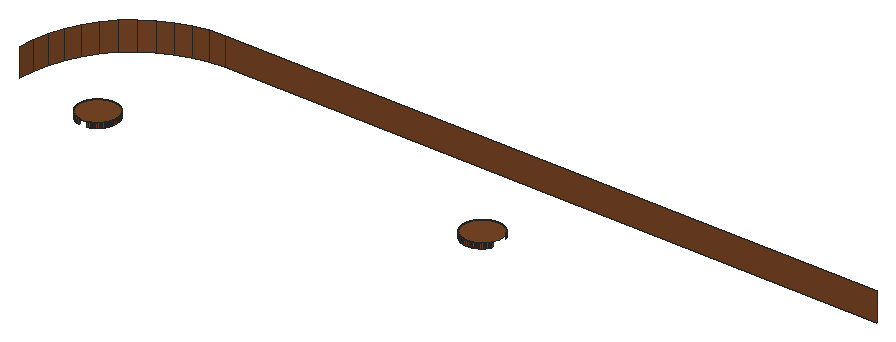
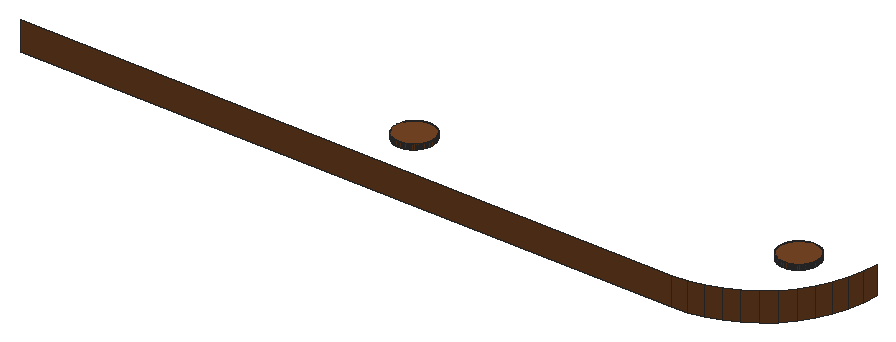
# SketchUp Ruby script. Lengths in inches.
U = 1.inch
M = Sketchup.active_model
def pt(a) = Geom::Point3d.new(a.map { |v| v * U })
def face(e, loops, mat)
  f = e.add_face(loops[0].map { |a| pt(a) })
  loops[1..].each { |l| e.add_face(l.map { |a| pt(a) }).erase! }
  f.material = f.back_material = mat if mat
  f
end
# faces: each face lists its corners as indices into pts; further lists are holes
def faces(e, pts, list, mat = nil) = list.each { |f| face(e, (f[0].is_a?(Array) ? f : [f]).map { |l| l.map { |i| pts[i] } }, mat) }
# xy, xz, yz: faces in a plane at the given z, y or x. An outline is a flat list of corners, or four numbers for a rectangle; further outlines are holes
def ring(l) = l.size == 4 ? [[l[0], l[1]], [l[2], l[1]], [l[2], l[3]], [l[0], l[3]]] : l.each_slice(2).to_a
def flat(e, list, mat, &to3) = list.each { |f| face(e, (f[0].is_a?(Array) ? f : [f]).map { |l| ring(l).map { |u, v| to3.(u, v) } }, mat) }
def xy(e, z, list, mat = nil) = flat(e, list, mat) { |x, y| [x, y, z] }
def xz(e, y, list, mat = nil) = flat(e, list, mat) { |x, z| [x, y, z] }
def yz(e, x, list, mat = nil) = flat(e, list, mat) { |y, z| [x, y, z] }
def lines(e, pts, list) = list.each { |a, b| e.add_line(pt(pts[a]), pt(pts[b])) }
# prism: a flat outline (further loops are holes) pulled along v
def prism(e, loops, v, mat = nil)
  f = face(e, loops, mat); d = Geom::Vector3d.new(v.map { |x| x * U })
  f.pushpull(f.normal.samedirection?(d) ? d.length : -d.length)
end
def box(e, o, s, mat = nil) = prism(e, [[o, [o[0] + s[0], o[1], o[2]], [o[0] + s[0], o[1] + s[1], o[2]], [o[0], o[1] + s[1], o[2]]]], [0, 0, s[2]], mat)
def at(x, y, z, deg = 0) = Geom::Transformation.translation(pt([x, y, z])) * Geom::Transformation.rotation(ORIGIN, Z_AXIS, deg.degrees)
def axes(o, x, y, z) = Geom::Transformation.new([*x, 0, *y, 0, *z, 0, *pt(o).to_a, 1])
def part(name) = M.definitions.add(name)
# library, detail: a bought-in or finely detailed component or shape, given as its bounding box
def library(name, o, s) = part(name).tap { |d| box(d.entities, o, s) }
def detail(e, o, s) = box(e.add_group.entities, o, s)
def put(e, d, t, mat = nil) = e.add_instance(d, t).tap { |i| i.material = mat if mat }
def group(e, t, mat = nil) = e.add_group.tap { |g| g.transformation = t; g.material = mat if mat }.entities
root = M.entities
M.materials.add("[Wood Veneer 01]3").color = [120, 70, 37]
xy(root,118.5,[[71.9,168,71.74,168.02,71.65,168.03,71.41,168.09,71.17,168.18,71.1,168.21,71.02,168.25,70.95,168.3,70.88,168.34,70.8125,168.39,70.75,168.44,70.68,168.5,70.62,168.55,70.5625,168.61,70.5,168.67,70.45,168.74,70.4,168.8,70.3,168.94,70.26,169.01,70.22,169.09,70.18,169.16,70.09,169.4,70.03,169.64,70.01,169.8,70,169.89,70,170.14,70.01,170.22,70.02,170.31,70.1,170.63,70.16,170.79,70.2,170.86,70.23,170.9375,70.27,171.01,70.47,171.29,70.52,171.35,70.64,171.47,70.7,171.52,70.77,171.58,70.84,171.625,70.9,171.67,70.98,171.72,71.05,171.76,71.125,171.8,71.2,171.83,71.44,171.92,71.6,171.96,71.68,171.97,71.76,171.99,71.85,171.99,71.93,172,72.1,172,72.26,171.98,72.35,171.97,72.59,171.91,72.83,171.82,72.9,171.79,72.98,171.75,73.05,171.7,73.12,171.66,73.1875,171.61,73.25,171.56,73.32,171.5,73.38,171.45,73.4375,171.39,73.5,171.33,73.55,171.26,73.6,171.2,73.7,171.06,73.74,170.99,73.78,170.91,73.82,170.84,73.91,170.6,73.97,170.36,73.99,170.2,74,170.11,74,169.86,73.99,169.78,73.98,169.69,73.9,169.37,73.84,169.21,73.8,169.14,73.77,169.0625,73.73,168.99,73.53,168.71,73.48,168.65,73.36,168.53,73.3,168.48,73.23,168.42,73.16,168.375,73.1,168.33,73.02,168.28,72.95,168.24,72.875,168.2,72.8,168.17,72.56,168.08,72.4,168.04,72.32,168.03,72.24,168.01,72.15,168.01,72.07,168],[109.4,172,109.24,172.02,109.15,172.03,108.91,172.09,108.67,172.18,108.6,172.21,108.52,172.25,108.45,172.3,108.38,172.34,108.3125,172.39,108.25,172.44,108.18,172.5,108.12,172.55,108.0625,172.61,108,172.67,107.95,172.74,107.9,172.8,107.8,172.94,107.76,173.01,107.72,173.09,107.68,173.16,107.59,173.4,107.53,173.64,107.51,173.8,107.5,173.89,107.5,174.14,107.51,174.22,107.52,174.31,107.6,174.63,107.66,174.79,107.7,174.86,107.73,174.9375,107.77,175.01,107.97,175.29,108.02,175.35,108.14,175.47,108.2,175.52,108.27,175.58,108.34,175.625,108.4,175.67,108.48,175.72,108.55,175.76,108.625,175.8,108.7,175.83,108.94,175.92,109.1,175.96,109.18,175.97,109.26,175.99,109.35,175.99,109.43,176,109.6,176,109.76,175.98,109.85,175.97,110.09,175.91,110.33,175.82,110.4,175.79,110.48,175.75,110.55,175.7,110.62,175.66,110.6875,175.61,110.75,175.56,110.82,175.5,110.88,175.45,110.9375,175.39,111,175.33,111.05,175.26,111.1,175.2,111.2,175.06,111.24,174.99,111.28,174.91,111.32,174.84,111.41,174.6,111.47,174.36,111.49,174.2,111.5,174.11,111.5,173.86,111.49,173.78,111.48,173.69,111.4,173.37,111.34,173.21,111.3,173.14,111.27,173.0625,111.23,172.99,111.03,172.71,110.98,172.65,110.86,172.53,110.8,172.48,110.73,172.42,110.66,172.375,110.6,172.33,110.52,172.28,110.45,172.24,110.375,172.2,110.3,172.17,110.06,172.08,109.9,172.04,109.82,172.03,109.74,172.01,109.65,172.01,109.57,172]],"[Wood Veneer 01]3")
xz(root,171.99,[[71.76,118,71.85,118.5]],"[Wood Veneer 01]3")
xz(root,172,[[71.93,118,72.01,118.5],[72.01,118,72.1,118.5],[109.4,118,109.49,118.5],[109.49,118,109.57,118.5]],"[Wood Veneer 01]3")
xz(root,172.01,[[109.65,118,109.74,118.5]],"[Wood Veneer 01]3")
xz(root,175.99,[[109.26,118,109.35,118.5]],"[Wood Veneer 01]3")
xz(root,176,[[109.43,118,109.51,118.5],[109.51,118,109.6,118.5]],"[Wood Veneer 01]3")
xz(root,183,[[75,118,144,121]],"[Wood Veneer 01]3")
yz(root,70,[[169.89,118,169.97,118.5],[169.97,118,170.06,118.5],[170.06,118,170.14,118.5]],"[Wood Veneer 01]3")
yz(root,74,[[169.86,118,169.94,118.5],[169.94,118,170.03,118.5],[170.03,118,170.11,118.5]],"[Wood Veneer 01]3")
yz(root,107.5,[[173.89,118,173.97,118.5],[173.97,118,174.06,118.5],[174.06,118,174.14,118.5]],"[Wood Veneer 01]3")
p = [[71.57,168.05,118],[71.49,168.07,118],[71.49,168.07,118.5],[71.57,168.05,118.5],[71.65,168.03,118],[71.65,168.03,118.5],
  [72.48,168.06,118],[72.4,168.04,118],[72.4,168.04,118.5],[72.48,168.06,118.5],[71.25,168.15,118],[71.17,168.18,118],
  [71.17,168.18,118.5],[71.25,168.15,118.5],[71.41,168.09,118],[71.33,168.12,118],[71.33,168.12,118.5],[71.41,168.09,118.5],
  [72.56,168.08,118],[72.56,168.08,118.5],[72.64,168.11,118],[72.64,168.11,118.5],[72.72,168.14,118],[72.72,168.14,118.5],
  [72.8,168.17,118],[72.8,168.17,118.5],[71.1,168.21,118],[71.02,168.25,118],[71.02,168.25,118.5],[71.1,168.21,118.5],
  [72.875,168.2,118],[72.875,168.2,118.5],[72.95,168.24,118],[72.95,168.24,118.5],[73.02,168.28,118],[73.02,168.28,118.5],
  [70.88,168.34,118],[70.8125,168.39,118],[70.8125,168.39,118.5],[70.88,168.34,118.5],[70.95,168.3,118],[70.95,168.3,118.5],
  [73.1,168.33,118],[73.1,168.33,118.5],[73.16,168.375,118],[73.16,168.375,118.5],[70.75,168.44,118],[70.75,168.44,118.5],
  [70.68,168.5,118],[70.68,168.5,118.5],[73.23,168.42,118],[73.23,168.42,118.5],[73.3,168.48,118],[73.3,168.48,118.5],
  [70.62,168.55,118],[70.62,168.55,118.5],[73.36,168.53,118],[73.36,168.53,118.5],[73.42,168.59,118],[73.42,168.59,118.5],
  [70.5625,168.61,118],[70.5,168.67,118],[70.5,168.67,118.5],[70.5625,168.61,118.5],[73.48,168.65,118],[73.48,168.65,118.5],
  [70.45,168.74,118],[70.4,168.8,118],[70.4,168.8,118.5],[70.45,168.74,118.5],[73.53,168.71,118],[73.53,168.71,118.5],
  [73.58,168.78,118],[73.58,168.78,118.5],[70.35,168.87,118],[70.35,168.87,118.5],[73.63,168.85,118],[73.63,168.85,118.5],
  [73.68,168.92,118],[73.68,168.92,118.5],[70.3,168.94,118],[70.3,168.94,118.5],[70.26,169.01,118],[70.26,169.01,118.5],
  [73.73,168.99,118],[73.73,168.99,118.5],[70.22,169.09,118],[70.22,169.09,118.5],[73.77,169.0625,118],[73.77,169.0625,118.5],
  [70.18,169.16,118],[70.18,169.16,118.5],[73.8,169.14,118],[73.8,169.14,118.5],[73.84,169.21,118],[73.84,169.21,118.5],
  [70.15,169.24,118],[70.12,169.32,118],[70.12,169.32,118.5],[70.15,169.24,118.5],[73.87,169.29,118],[73.87,169.29,118.5],
  [70.09,169.4,118],[70.09,169.4,118.5],[73.9,169.37,118],[73.9,169.37,118.5],[70.07,169.48,118],[70.07,169.48,118.5],
  [73.92,169.45,118],[73.92,169.45,118.5],[73.94,169.53,118],[73.94,169.53,118.5],[70.05,169.56,118],[70.05,169.56,118.5],
  [73.96,169.61,118],[73.96,169.61,118.5],[70.03,169.64,118],[70.03,169.64,118.5],[70.02,169.72,118],[70.02,169.72,118.5],
  [73.98,169.69,118],[73.98,169.69,118.5],[70.01,169.8,118],[70.01,169.8,118.5],[73.99,169.78,118],[73.99,169.78,118.5],
  [70,169.89,118],[70,169.89,118.5],[74,169.86,118],[74,169.86,118.5],[70,170.14,118],[70.01,170.22,118],
  [70.01,170.22,118.5],[70,170.14,118.5],[73.99,170.2,118],[74,170.11,118],[74,170.11,118.5],[73.99,170.2,118.5],
  [70.02,170.31,118],[70.02,170.31,118.5],[73.98,170.28,118],[73.98,170.28,118.5],[70.04,170.39,118],[70.04,170.39,118.5],
  [73.97,170.36,118],[73.97,170.36,118.5],[70.06,170.47,118],[70.06,170.47,118.5],[73.93,170.52,118],[73.95,170.44,118],
  [73.95,170.44,118.5],[73.93,170.52,118.5],[70.08,170.55,118],[70.08,170.55,118.5],[73.91,170.6,118],[73.91,170.6,118.5],
  [70.1,170.63,118],[70.1,170.63,118.5],[70.13,170.71,118],[70.13,170.71,118.5],[73.88,170.68,118],[73.88,170.68,118.5],
  [70.16,170.79,118],[70.16,170.79,118.5],[73.85,170.76,118],[73.85,170.76,118.5],[70.2,170.86,118],[70.2,170.86,118.5],
  [73.82,170.84,118],[73.82,170.84,118.5],[73.78,170.91,118],[73.78,170.91,118.5],[70.23,170.9375,118],[70.23,170.9375,118.5],
  [70.27,171.01,118],[70.27,171.01,118.5],[73.74,170.99,118],[73.74,170.99,118.5],[63,171,121],[63.1,172.57,121],
  [63.1,172.57,118],[63,171,118],[70.32,171.08,118],[70.32,171.08,118.5],[73.7,171.06,118],[73.7,171.06,118.5],
  [70.37,171.15,118],[70.37,171.15,118.5],[73.6,171.2,118],[73.65,171.13,118],[73.65,171.13,118.5],[73.6,171.2,118.5],
  [70.42,171.22,118],[70.42,171.22,118.5],[70.47,171.29,118],[70.47,171.29,118.5],[73.55,171.26,118],[73.55,171.26,118.5],
  [70.52,171.35,118],[70.52,171.35,118.5],[70.58,171.41,118],[70.58,171.41,118.5],[73.4375,171.39,118],[73.5,171.33,118],
  [73.5,171.33,118.5],[73.4375,171.39,118.5],[70.64,171.47,118],[70.64,171.47,118.5],[73.32,171.5,118],[73.38,171.45,118],
  [73.38,171.45,118.5],[73.32,171.5,118.5],[70.7,171.52,118],[70.7,171.52,118.5],[70.77,171.58,118],[70.77,171.58,118.5],
  [73.25,171.56,118],[73.25,171.56,118.5],[70.84,171.625,118],[70.84,171.625,118.5],[70.9,171.67,118],[70.9,171.67,118.5],
  [73.12,171.66,118],[73.1875,171.61,118],[73.1875,171.61,118.5],[73.12,171.66,118.5],[70.98,171.72,118],[70.98,171.72,118.5],
  [71.05,171.76,118],[71.05,171.76,118.5],[72.9,171.79,118],[72.98,171.75,118],[72.98,171.75,118.5],[72.9,171.79,118.5],
  [73.05,171.7,118],[73.05,171.7,118.5],[71.125,171.8,118],[71.125,171.8,118.5],[71.2,171.83,118],[71.2,171.83,118.5],
  [71.28,171.86,118],[71.28,171.86,118.5],[72.75,171.85,118],[72.83,171.82,118],[72.83,171.82,118.5],[72.75,171.85,118.5],
  [71.36,171.89,118],[71.36,171.89,118.5],[71.44,171.92,118],[71.44,171.92,118.5],[71.52,171.94,118],[71.52,171.94,118.5],
  [71.6,171.96,118],[71.6,171.96,118.5],[72.43,171.95,118],[72.51,171.93,118],[72.51,171.93,118.5],[72.43,171.95,118.5],
  [72.59,171.91,118],[72.59,171.91,118.5],[72.67,171.88,118],[72.67,171.88,118.5],[71.68,171.97,118],[71.68,171.97,118.5],
  [71.76,171.99,118],[71.76,171.99,118.5],[71.85,171.99,118],[71.93,172,118],[71.93,172,118.5],[71.85,171.99,118.5],
  [72.1,172,118],[72.18,171.99,118],[72.18,171.99,118.5],[72.1,172,118.5],[72.26,171.98,118],[72.26,171.98,118.5],
  [72.35,171.97,118],[72.35,171.97,118.5],[109.07,172.05,118],[108.99,172.07,118],[108.99,172.07,118.5],[109.07,172.05,118.5],
  [109.15,172.03,118],[109.15,172.03,118.5],[109.32,172.01,118],[109.24,172.02,118],[109.24,172.02,118.5],[109.32,172.01,118.5],
  [109.4,172,118],[109.4,172,118.5],[109.65,172.01,118],[109.57,172,118],[109.57,172,118.5],[109.65,172.01,118.5],
  [109.82,172.03,118],[109.74,172.01,118],[109.74,172.01,118.5],[109.82,172.03,118.5],[109.9,172.04,118],[109.9,172.04,118.5],
  [109.98,172.06,118],[109.98,172.06,118.5],[108.75,172.15,118],[108.67,172.18,118],[108.67,172.18,118.5],[108.75,172.15,118.5],
  [108.91,172.09,118],[108.83,172.12,118],[108.83,172.12,118.5],[108.91,172.09,118.5],[110.06,172.08,118],[110.06,172.08,118.5],
  [110.14,172.11,118],[110.14,172.11,118.5],[110.22,172.14,118],[110.22,172.14,118.5],[110.3,172.17,118],[110.3,172.17,118.5],
  [108.6,172.21,118],[108.52,172.25,118],[108.52,172.25,118.5],[108.6,172.21,118.5],[110.375,172.2,118],[110.375,172.2,118.5],
  [110.45,172.24,118],[110.45,172.24,118.5],[110.52,172.28,118],[110.52,172.28,118.5],[108.38,172.34,118],[108.3125,172.39,118],
  [108.3125,172.39,118.5],[108.38,172.34,118.5],[108.45,172.3,118],[108.45,172.3,118.5],[110.6,172.33,118],[110.6,172.33,118.5],
  [110.66,172.375,118],[110.66,172.375,118.5],[108.25,172.44,118],[108.25,172.44,118.5],[108.18,172.5,118],[108.18,172.5,118.5],
  [110.73,172.42,118],[110.73,172.42,118.5],[110.8,172.48,118],[110.8,172.48,118.5],[108.12,172.55,118],[108.12,172.55,118.5],
  [110.86,172.53,118],[110.86,172.53,118.5],[110.92,172.59,118],[110.92,172.59,118.5],[63.41,174.11,121],[63.41,174.11,118],
  [108.0625,172.61,118],[108,172.67,118],[108,172.67,118.5],[108.0625,172.61,118.5],[110.98,172.65,118],[110.98,172.65,118.5],
  [107.95,172.74,118],[107.9,172.8,118],[107.9,172.8,118.5],[107.95,172.74,118.5],[111.03,172.71,118],[111.03,172.71,118.5],
  [111.08,172.78,118],[111.08,172.78,118.5],[107.85,172.87,118],[107.85,172.87,118.5],[111.13,172.85,118],[111.13,172.85,118.5],
  [111.18,172.92,118],[111.18,172.92,118.5],[107.8,172.94,118],[107.8,172.94,118.5],[107.76,173.01,118],[107.76,173.01,118.5],
  [111.23,172.99,118],[111.23,172.99,118.5],[107.72,173.09,118],[107.72,173.09,118.5],[111.27,173.0625,118],[111.27,173.0625,118.5],
  [107.68,173.16,118],[107.68,173.16,118.5],[111.3,173.14,118],[111.3,173.14,118.5],[107.65,173.24,118],[107.62,173.32,118],
  [107.62,173.32,118.5],[107.65,173.24,118.5],[107.59,173.4,118],[107.59,173.4,118.5],[107.57,173.48,118],[107.57,173.48,118.5],
  [107.55,173.56,118],[107.55,173.56,118.5],[107.53,173.64,118],[107.53,173.64,118.5],[107.52,173.72,118],[107.52,173.72,118.5],
  [107.51,173.8,118],[107.51,173.8,118.5],[107.5,173.89,118],[107.5,173.89,118.5],[63.91,175.59,121],[63.91,175.59,118],
  [107.5,174.14,118],[107.51,174.22,118],[107.51,174.22,118.5],[107.5,174.14,118.5],[107.52,174.31,118],[107.52,174.31,118.5],
  [107.54,174.39,118],[107.54,174.39,118.5],[107.56,174.47,118],[107.56,174.47,118.5],[107.58,174.55,118],[107.58,174.55,118.5],
  [107.6,174.63,118],[107.6,174.63,118.5],[107.63,174.71,118],[107.63,174.71,118.5],[107.66,174.79,118],[107.66,174.79,118.5],
  [107.7,174.86,118],[107.7,174.86,118.5],[107.73,174.9375,118],[107.73,174.9375,118.5],[107.77,175.01,118],[107.77,175.01,118.5],
  [111.24,174.99,118],[111.28,174.91,118],[111.28,174.91,118.5],[111.24,174.99,118.5],[107.82,175.08,118],[107.82,175.08,118.5],
  [111.2,175.06,118],[111.2,175.06,118.5],[107.87,175.15,118],[107.87,175.15,118.5],[111.1,175.2,118],[111.15,175.13,118],
  [111.15,175.13,118.5],[111.1,175.2,118.5],[107.92,175.22,118],[107.92,175.22,118.5],[107.97,175.29,118],[107.97,175.29,118.5],
  [111.05,175.26,118],[111.05,175.26,118.5],[108.02,175.35,118],[108.02,175.35,118.5],[108.08,175.41,118],[108.08,175.41,118.5],
  [110.9375,175.39,118],[111,175.33,118],[111,175.33,118.5],[110.9375,175.39,118.5],[108.14,175.47,118],[108.14,175.47,118.5],
  [110.82,175.5,118],[110.88,175.45,118],[110.88,175.45,118.5],[110.82,175.5,118.5],[108.2,175.52,118],[108.2,175.52,118.5],
  [108.27,175.58,118],[108.27,175.58,118.5],[110.75,175.56,118],[110.75,175.56,118.5],[64.61,177,121],[64.61,177,118],
  [108.34,175.625,118],[108.34,175.625,118.5],[108.4,175.67,118],[108.4,175.67,118.5],[110.62,175.66,118],[110.6875,175.61,118],
  [110.6875,175.61,118.5],[110.62,175.66,118.5],[108.48,175.72,118],[108.48,175.72,118.5],[108.55,175.76,118],[108.55,175.76,118.5],
  [110.4,175.79,118],[110.48,175.75,118],[110.48,175.75,118.5],[110.4,175.79,118.5],[110.55,175.7,118],[110.55,175.7,118.5],
  [108.625,175.8,118],[108.625,175.8,118.5],[108.7,175.83,118],[108.7,175.83,118.5],[108.78,175.86,118],[108.78,175.86,118.5],
  [110.25,175.85,118],[110.33,175.82,118],[110.33,175.82,118.5],[110.25,175.85,118.5],[108.86,175.89,118],[108.86,175.89,118.5],
  [108.94,175.92,118],[108.94,175.92,118.5],[109.02,175.94,118],[109.02,175.94,118.5],[109.1,175.96,118],[109.1,175.96,118.5],
  [109.93,175.95,118],[110.01,175.93,118],[110.01,175.93,118.5],[109.93,175.95,118.5],[110.09,175.91,118],[110.09,175.91,118.5],
  [110.17,175.88,118],[110.17,175.88,118.5],[109.18,175.97,118],[109.18,175.97,118.5],[109.26,175.99,118],[109.26,175.99,118.5],
  [109.35,175.99,118],[109.43,176,118],[109.43,176,118.5],[109.35,175.99,118.5],[109.6,176,118],[109.68,175.99,118],
  [109.68,175.99,118.5],[109.6,176,118.5],[109.76,175.98,118],[109.76,175.98,118.5],[109.85,175.97,118],[109.85,175.97,118.5],
  [65.48,178.31,121],[65.48,178.31,118],[66.51,179.49,121],[66.51,179.49,118],[67.69,180.52,121],[67.69,180.52,118],
  [69,181.39,121],[69,181.39,118],[70.41,182.09,121],[70.41,182.09,118],[71.89,182.59,121],[71.89,182.59,118],
  [73.43,182.9,121],[73.43,182.9,118],[75,183,121],[75,183,118]]
faces(root,p,[[0,1,2,3],[4,0,3,5],[6,7,8,9],[10,11,12,13],[14,15,16,17],[15,10,13,16],[1,14,17,2],[18,6,9,19],
  [20,18,19,21],[22,20,21,23],[24,22,23,25],[26,27,28,29],[11,26,29,12],[30,24,25,31],[32,30,31,33],[34,32,33,35],
  [36,37,38,39],[40,36,39,41],[27,40,41,28],[42,34,35,43],[44,42,43,45],[37,46,47,38],[46,48,49,47],[50,44,45,51],
  [52,50,51,53],[48,54,55,49],[56,52,53,57],[58,56,57,59],[60,61,62,63],[54,60,63,55],[64,58,59,65],[66,67,68,69],
  [61,66,69,62],[70,64,65,71],[72,70,71,73],[67,74,75,68],[76,72,73,77],[78,76,77,79],[74,80,81,75],[80,82,83,81],
  [84,78,79,85],[82,86,87,83],[88,84,85,89],[86,90,91,87],[92,88,89,93],[94,92,93,95],[96,97,98,99],[90,96,99,91],
  [100,94,95,101],[97,102,103,98],[104,100,101,105],[102,106,107,103],[108,104,105,109],[110,108,109,111],[106,112,113,107],[114,110,111,115],
  [112,116,117,113],[116,118,119,117],[120,114,115,121],[118,122,123,119],[124,120,121,125],[122,126,127,123],[128,124,125,129],[130,131,132,133],
  [134,135,136,137],[131,138,139,132],[140,134,137,141],[138,142,143,139],[144,140,141,145],[142,146,147,143],[148,149,150,151],[149,144,145,150],
  [146,152,153,147],[154,148,151,155],[152,156,157,153],[156,158,159,157],[160,154,155,161],[158,162,163,159],[164,160,161,165],[162,166,167,163],
  [168,164,165,169],[170,168,169,171],[166,172,173,167],[172,174,175,173],[176,170,171,177],[178,179,180,181],[174,182,183,175],[184,176,177,185],
  [182,186,187,183],[188,189,190,191],[189,184,185,190],[186,192,193,187],[192,194,195,193],[196,188,191,197],[194,198,199,195],[198,200,201,199],
  [202,203,204,205],[203,196,197,204],[200,206,207,201],[208,209,210,211],[209,202,205,210],[206,212,213,207],[212,214,215,213],[216,208,211,217],
  [214,218,219,215],[218,220,221,219],[222,223,224,225],[223,216,217,224],[220,226,227,221],[226,228,229,227],[230,231,232,233],[234,222,225,235],
  [231,234,235,232],[228,236,237,229],[236,238,239,237],[238,240,241,239],[242,243,244,245],[243,230,233,244],[240,246,247,241],[246,248,249,247],
  [248,250,251,249],[250,252,253,251],[254,255,256,257],[255,258,259,256],[258,260,261,259],[260,242,245,261],[252,262,263,253],[262,264,265,263],
  [266,267,268,269],[270,271,272,273],[271,274,275,272],[276,254,257,277],[274,276,277,275],[278,279,280,281],[282,278,281,283],[284,285,286,287],
  [285,282,283,286],[288,284,287,289],[290,291,292,293],[294,295,296,297],[298,294,297,299],[300,298,299,301],[302,303,304,305],[306,307,308,309],
  [307,302,305,308],[279,306,309,280],[310,300,301,311],[312,310,311,313],[314,312,313,315],[316,314,315,317],[318,319,320,321],[303,318,321,304],
  [322,316,317,323],[324,322,323,325],[326,324,325,327],[328,329,330,331],[332,328,331,333],[319,332,333,320],[334,326,327,335],[336,334,335,337],
  [329,338,339,330],[338,340,341,339],[342,336,337,343],[344,342,343,345],[340,346,347,341],[348,344,345,349],[350,348,349,351],[179,352,353,180],
  [354,355,356,357],[346,354,357,347],[358,350,351,359],[360,361,362,363],[355,360,363,356],[364,358,359,365],[366,364,365,367],[361,368,369,362],
  [370,366,367,371],[372,370,371,373],[368,374,375,369],[374,376,377,375],[378,372,373,379],[376,380,381,377],[382,378,379,383],[380,384,385,381],
  [386,382,383,387],[388,389,390,391],[384,388,391,385],[389,392,393,390],[392,394,395,393],[394,396,397,395],[396,398,399,397],[398,400,401,399],
  [400,402,403,401],[402,404,405,403],[352,406,407,353],[408,409,410,411],[409,412,413,410],[412,414,415,413],[414,416,417,415],[416,418,419,417],
  [418,420,421,419],[420,422,423,421],[422,424,425,423],[424,426,427,425],[426,428,429,427],[428,430,431,429],[432,433,434,435],[430,436,437,431],
  [438,432,435,439],[436,440,441,437],[442,443,444,445],[443,438,439,444],[440,446,447,441],[446,448,449,447],[450,442,445,451],[448,452,453,449],
  [452,454,455,453],[456,457,458,459],[457,450,451,458],[454,460,461,455],[462,463,464,465],[463,456,459,464],[460,466,467,461],[466,468,469,467],
  [470,462,465,471],[406,472,473,407],[468,474,475,469],[474,476,477,475],[478,479,480,481],[479,470,471,480],[476,482,483,477],[482,484,485,483],
  [486,487,488,489],[490,478,481,491],[487,490,491,488],[484,492,493,485],[492,494,495,493],[494,496,497,495],[498,499,500,501],[499,486,489,500],
  [496,502,503,497],[502,504,505,503],[504,506,507,505],[506,508,509,507],[510,511,512,513],[511,514,515,512],[514,516,517,515],[516,498,501,517],
  [508,518,519,509],[518,520,521,519],[522,523,524,525],[526,527,528,529],[527,530,531,528],[532,510,513,533],[530,532,533,531],[472,534,535,473],
  [534,536,537,535],[536,538,539,537],[538,540,541,539],[540,542,543,541],[542,544,545,543],[544,546,547,545],[546,548,549,547]],"[Wood Veneer 01]3")
